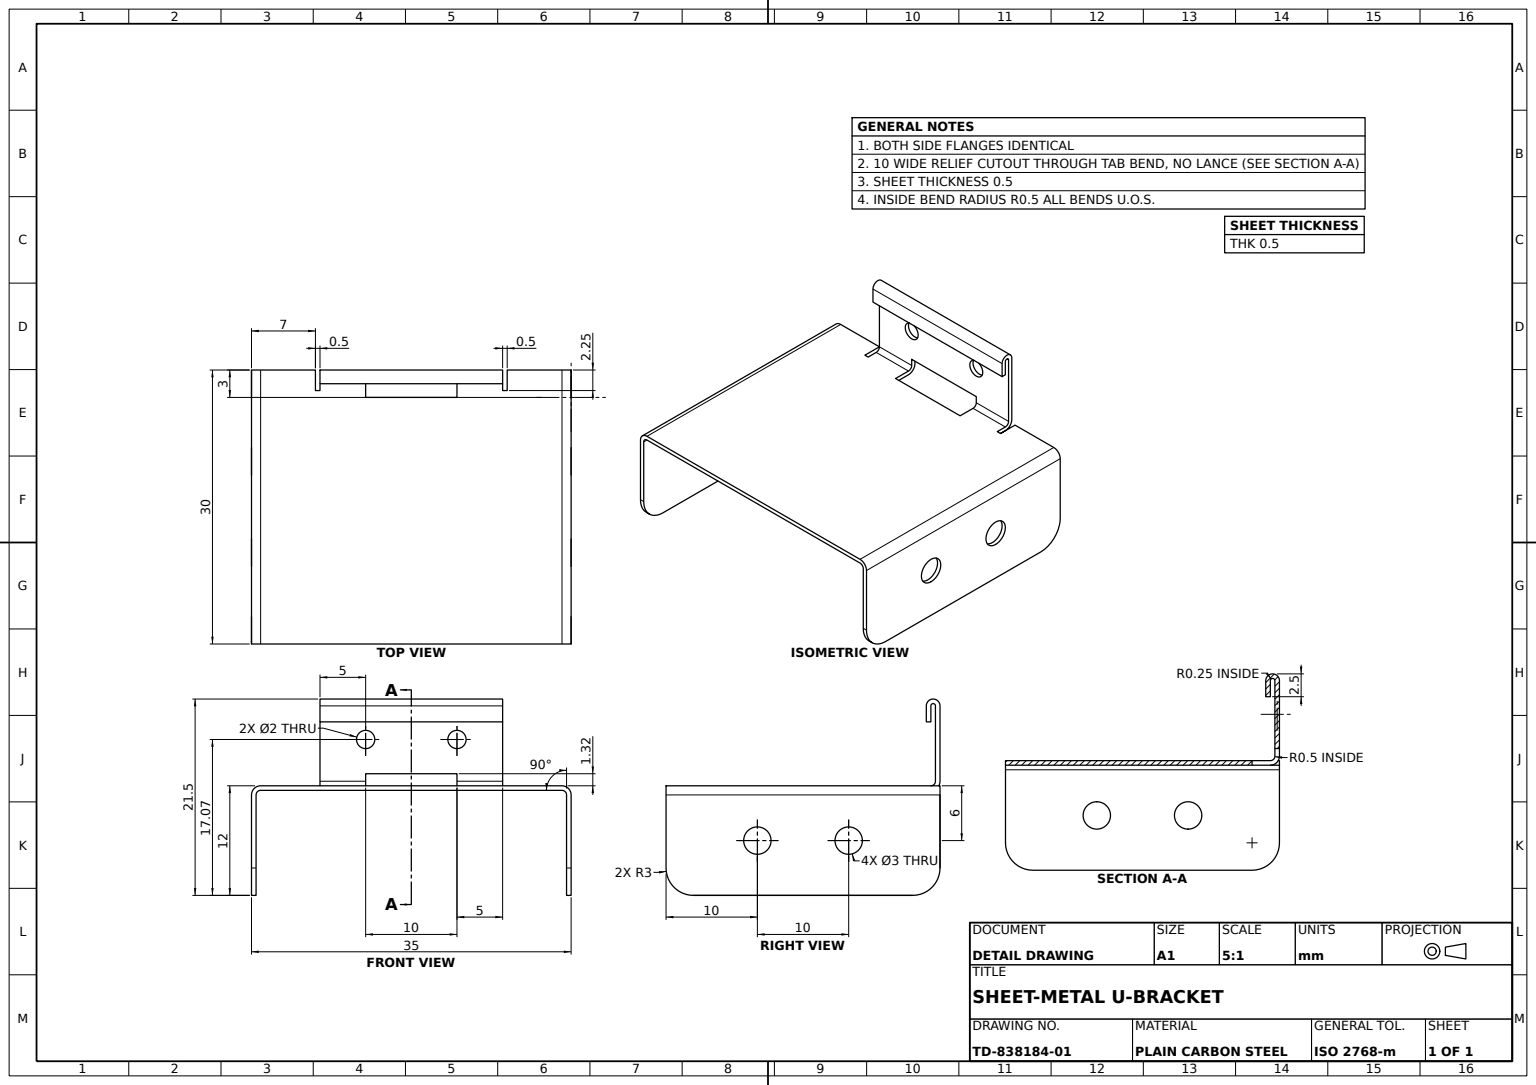
solid
v1 (-17.5,-1,-15)
v2 (-17.5,-9,-15)
e1 v1 v2 LINE
v3 (-17,-1,-15)
e2 v3 v1 LINE
v4 (-17,-9,-15)
e3 v3 v4 LINE
e4 v4 v2 LINE
face PLANE(AX(P(-17.5,-12,-15),D(0,0,1),D(1,0,0))) rev [-e1 -e2 e3 e4]
v5 (17.5,-9,-15)
v6 (17,-9,-15)
e5 v5 v6 LINE
v7 (17,-1,-15)
e6 v6 v7 LINE
v8 (17.5,-1,-15)
e7 v7 v8 LINE
e8 v5 v8 LINE
face PLANE(AX(P(17.5,-0.5,-15),D(0,0,1),D(1,0,0))) rev [e5 e6 e7 -e8]
v9 (-10,0,-12.75)
v10 (-10,-0.5,-12.75)
e9 v9 v10 LINE
v11 (-10,0,-14)
e10 v9 v11 LINE
v12 (-10,-0.5,-14)
e11 v11 v12 LINE
e12 v10 v12 LINE
face PLANE(AX(P(-10,0,-12.75),D(-1,0,0),D(0,0,1))) [-e9 e10 e11 -e12]
v13 (-5,1.321903,-15)
v14 (-5,0.5,-15)
e13 v13 v14 LINE
v15 (-5,1.321903,-14.5)
e14 v13 v15 LINE
v16 (-5,0.5,-14.5)
e15 v15 v16 LINE
e16 v14 v16 LINE
face PLANE(AX(P(-5,-2.678097,-15),D(-1,0,0),D(0,-1,0))) rev [-e13 e14 e15 -e16]
v17 (-10,0.5,-14.5)
v18 (-10,8.75,-14.5)
e17 v17 v18 LINE
v19 (-10,8.75,-15)
e18 v18 v19 LINE
v20 (-10,0.5,-15)
e19 v20 v19 LINE
e20 v17 v20 LINE
face PLANE(AX(P(-10,9.5,-15),D(1,0,0),D(0,0,-1))) rev [e17 e18 -e19 -e20]
v21 (16.5,-0.5,-15)
e21 v21 v7 CIRCLE(AX(P(16.5,-1,-15),D(0,0,-1),D(-1,0,0)),0.5)
v22 (17,-1,15)
e22 v7 v22 LINE
v23 (16.5,-0.5,15)
e23 v22 v23 CIRCLE(AX(P(16.5,-1,15),D(0,0,1),D(1,0,0)),0.5)
e24 v23 v21 LINE
face CYL(AX(P(16.5,-1,-30.027286),D(0,0,1),D(1,0,0)),0.5) rev [e21 e22 e23 e24]
v24 (5,4.070796,-15)
v25 (5,4.070796,-14.5)
e25 v24 v25 LINE
v26 (5,6.070796,-14.5)
e26 v25 v26 CIRCLE(AX(P(5,5.070796,-14.5),D(0,0,1),D(0,1,0)),1)
v27 (5,6.070796,-15)
e27 v27 v26 LINE
e28 v24 v27 CIRCLE(AX(P(5,5.070796,-15),D(0,0,1),D(0,1,0)),1)
face CYL(AX(P(5,5.070796,-15),D(0,0,1),D(0,-1,0)),1) rev [e25 e26 -e27 -e28]
v28 (5,1.321903,-15)
e29 v28 v13 LINE
v29 (5,1.321903,-14.5)
e30 v28 v29 LINE
e31 v29 v15 LINE
face PLANE(AX(P(-5,1.321903,-15),D(0,1,0),D(-1,0,0))) rev [-e14 -e29 e30 e31]
v30 (17,-7.5,5)
v31 (17.5,-7.5,5)
e32 v30 v31 LINE
v32 (17,-4.5,5)
e33 v30 v32 CIRCLE(AX(P(17,-6,5),D(-1,0,0),D(0,-1,0)),1.5)
v33 (17.5,-4.5,5)
e34 v32 v33 LINE
e35 v33 v31 CIRCLE(AX(P(17.5,-6,5),D(1,0,0),D(0,-1,0)),1.5)
face CYL(AX(P(-17.5,-6,5),D(1,0,0),D(0,1,0)),1.5) rev [-e32 e33 e34 e35]
v34 (-5,-0.5,-14)
e36 v14 v34 CIRCLE(AX(P(-5,0.5,-14),D(-1,0,0),D(0,0,1)),1)
e37 v12 v34 LINE
e38 v12 v20 CIRCLE(AX(P(-10,0.5,-14),D(1,0,0),D(0,0,-1)),1)
e39 v20 v14 LINE
face CYL(AX(P(-12.661193,0.5,-14),D(1,0,0),D(0,1,0)),1) [e36 -e37 e38 e39]
v35 (16.5,0,-15)
e40 v21 v35 LINE
e41 v35 v8 CIRCLE(AX(P(16.5,-1,-15),D(0,0,-1),D(1,0,0)),1)
face PLANE(AX(P(16.5,-1,-15),D(0,0,1),D(1,0,0))) rev [-e21 e40 e41 -e7]
e42 v11 v17 CIRCLE(AX(P(-10,0.5,-14),D(1,0,0),D(0,1,0)),0.5)
face PLANE(AX(P(-10,0.5,-14),D(-1,0,0),D(0,0,1))) [-e38 -e11 e42 e20]
v36 (16.5,0,15)
e43 v23 v36 LINE
v37 (17.5,-1,15)
e44 v22 v37 LINE
e45 v37 v36 CIRCLE(AX(P(16.5,-1,15),D(0,0,1),D(1,0,0)),1)
face PLANE(AX(P(16.5,-1,15),D(0,0,-1),D(-1,0,0))) rev [-e43 -e23 e44 e45]
v38 (10,-0.5,-12.75)
v39 (10.5,-0.5,-12.75)
e46 v38 v39 LINE
v40 (10,0,-12.75)
e47 v40 v38 LINE
v41 (10.5,0,-12.75)
e48 v40 v41 LINE
e49 v41 v39 LINE
face PLANE(AX(P(10,0,-12.75),D(0,0,-1),D(0,1,0))) [-e46 -e47 e48 e49]
v42 (-10.5,0,-15)
v43 (-10.5,-0.5,-15)
e50 v42 v43 LINE
v44 (-16.5,-0.5,-15)
e51 v43 v44 LINE
v45 (-16.5,0,-15)
e52 v44 v45 LINE
e53 v42 v45 LINE
face PLANE(AX(P(-17.5,-0.5,-15),D(0,0,-1),D(-1,0,0))) [e50 e51 e52 -e53]
v46 (10,8.75,-13.5)
v47 (10,7,-13.5)
e54 v46 v47 LINE
v48 (-10,8.75,-13.5)
e55 v48 v46 LINE
v49 (-10,7,-13.5)
e56 v49 v48 LINE
e57 v47 v49 LINE
face PLANE(AX(P(0,7.875,-13.5),D(0,0,1),D(0,-1,0))) [-e54 -e55 -e56 -e57]
v50 (10,7,-14)
v51 (-10,7,-14)
e58 v50 v51 LINE
v52 (-10,8.75,-14)
e59 v51 v52 LINE
v53 (10,8.75,-14)
e60 v52 v53 LINE
e61 v53 v50 LINE
face PLANE(AX(P(0,7.875,-14),D(0,0,1),D(0,-1,0))) rev [e58 e59 e60 e61]
v54 (10,0,-14)
v55 (10,-0.5,-14)
e62 v54 v55 LINE
e63 v54 v40 LINE
e64 v55 v38 LINE
face PLANE(AX(P(10,0,-14),D(1,0,0),D(0,0,-1))) [-e62 e63 e47 -e64]
v56 (5,0,-14)
e65 v56 v54 LINE
v57 (5,0,-12)
e66 v57 v56 LINE
v58 (-5,0,-12)
e67 v58 v57 LINE
v59 (-5,0,-14)
e68 v59 v58 LINE
e69 v11 v59 LINE
v60 (-10.5,0,-12.75)
e70 v60 v9 LINE
e71 v42 v60 LINE
v61 (-16.5,0,15)
e72 v45 v61 LINE
e73 v61 v36 LINE
e74 v36 v35 LINE
v62 (10.5,0,-15)
e75 v35 v62 LINE
e76 v41 v62 LINE
face PLANE(AX(P(0,0,0),D(0,-1,0),D(0,0,-1))) rev [-e63 -e65 -e66 -e67 -e68 -e69 -e10 -e70 -e71 e53 e72 e73 e74 e75 -e76 -e48]
v63 (-17.5,-9,15)
v64 (-17,-9,15)
e77 v63 v64 LINE
v65 (-17.5,-12,12)
e78 v65 v63 CIRCLE(AX(P(-17.5,-9,12),D(-1,0,0),D(0,1,0)),3)
v66 (-17,-12,12)
e79 v66 v65 LINE
e80 v64 v66 CIRCLE(AX(P(-17,-9,12),D(1,0,0),D(0,1,0)),3)
face CYL(AX(P(-17.5,-9,12),D(1,0,0),D(0,1,0)),3) [-e77 -e78 -e79 -e80]
v67 (17.5,-7.5,-5)
v68 (17.5,-4.5,-5)
e81 v67 v68 CIRCLE(AX(P(17.5,-6,-5),D(1,0,0),D(0,1,0)),1.5)
v69 (17,-4.5,-5)
e82 v69 v68 LINE
v70 (17,-7.5,-5)
e83 v69 v70 CIRCLE(AX(P(17,-6,-5),D(-1,0,0),D(0,-1,0)),1.5)
e84 v70 v67 LINE
face CYL(AX(P(-17.5,-6,-5),D(1,0,0),D(0,1,0)),1.5) rev [e81 -e82 e83 e84]
v71 (-5,-0.5,-12)
v72 (5,-0.5,-12)
e85 v71 v72 LINE
e86 v71 v58 LINE
e87 v72 v57 LINE
face PLANE(AX(P(-5,-0.5,-12),D(0,0,1),D(1,0,0))) rev [-e85 e86 e67 -e87]
v73 (-10.5,-0.5,-12.75)
e88 v73 v10 LINE
e89 v60 v73 LINE
face PLANE(AX(P(-10.5,0,-12.75),D(0,0,-1),D(0,1,0))) [e9 -e88 -e89 e70]
e90 v32 v30 CIRCLE(AX(P(17,-6,5),D(-1,0,0),D(0,-1,0)),1.5)
e91 v31 v33 CIRCLE(AX(P(17.5,-6,5),D(1,0,0),D(0,-1,0)),1.5)
face CYL(AX(P(-17.5,-6,5),D(1,0,0),D(0,1,0)),1.5) rev [-e34 e90 e32 e91]
e92 v26 v25 CIRCLE(AX(P(5,5.070796,-14.5),D(0,0,1),D(0,1,0)),1)
e93 v27 v24 CIRCLE(AX(P(5,5.070796,-15),D(0,0,1),D(0,1,0)),1)
face CYL(AX(P(5,5.070796,-15),D(0,0,1),D(0,-1,0)),1) rev [e27 e92 -e25 -e93]
v74 (-5,4.070796,-15)
v75 (-5,6.070796,-15)
e94 v74 v75 CIRCLE(AX(P(-5,5.070796,-15),D(0,0,1),D(0,-1,0)),1)
v76 (-5,4.070796,-14.5)
e95 v74 v76 LINE
v77 (-5,6.070796,-14.5)
e96 v76 v77 CIRCLE(AX(P(-5,5.070796,-14.5),D(0,0,1),D(0,-1,0)),1)
e97 v75 v77 LINE
face CYL(AX(P(-5,5.070796,-15),D(0,0,1),D(0,-1,0)),1) rev [-e94 e95 e96 -e97]
e98 v77 v76 CIRCLE(AX(P(-5,5.070796,-14.5),D(0,0,1),D(0,-1,0)),1)
v78 (5,0.5,-14.5)
e99 v78 v29 LINE
v79 (10,0.5,-14.5)
e100 v79 v78 LINE
v80 (10,8.75,-14.5)
e101 v80 v79 LINE
e102 v18 v80 LINE
e103 v16 v17 LINE
face PLANE(AX(P(0,0,-14.5),D(0,0,1),D(0,-1,0))) [-e92 -e26] [-e96 -e98] [-e99 -e100 -e101 -e102 -e17 -e103 -e15 -e31]
v81 (17,-12,12)
v82 (17,-9,15)
e104 v81 v82 CIRCLE(AX(P(17,-9,12),D(-1,0,0),D(0,-1,0)),3)
e105 v22 v82 LINE
v83 (17,-12,-12)
e106 v6 v83 CIRCLE(AX(P(17,-9,-12),D(-1,0,0),D(0,-1,0)),3)
e107 v81 v83 LINE
e108 v70 v69 CIRCLE(AX(P(17,-6,-5),D(-1,0,0),D(0,-1,0)),1.5)
face PLANE(AX(P(17,0,0),D(-1,0,0),D(0,-1,0))) [e104 -e105 -e22 -e6 e106 -e107] [-e108 -e83] [-e90 -e33]
v84 (10.5,-0.5,-15)
e109 v21 v84 LINE
e110 v62 v84 LINE
face PLANE(AX(P(-17.5,-0.5,-15),D(0,0,-1),D(-1,0,0))) [-e75 -e40 e109 -e110]
e111 v75 v74 CIRCLE(AX(P(-5,5.070796,-15),D(0,0,1),D(0,-1,0)),1)
face CYL(AX(P(-5,5.070796,-15),D(0,0,1),D(0,-1,0)),1) rev [-e95 -e111 e97 e98]
v85 (5,-0.5,-14)
v86 (5,0.5,-15)
e112 v85 v86 CIRCLE(AX(P(5,0.5,-14),D(1,0,0),D(0,0,-1)),1)
e113 v85 v56 LINE
e114 v56 v78 CIRCLE(AX(P(5,0.5,-14),D(1,0,0),D(0,1,0)),0.5)
e115 v78 v86 LINE
face PLANE(AX(P(5,0.5,-14),D(-1,0,0),D(0,0,1))) [-e112 e113 e114 e115]
v87 (-17.5,-4.5,-5)
v88 (-17.5,-7.5,-5)
e116 v87 v88 CIRCLE(AX(P(-17.5,-6,-5),D(1,0,0),D(0,1,0)),1.5)
v89 (-17,-4.5,-5)
e117 v87 v89 LINE
v90 (-17,-7.5,-5)
e118 v89 v90 CIRCLE(AX(P(-17,-6,-5),D(1,0,0),D(0,1,0)),1.5)
e119 v88 v90 LINE
face CYL(AX(P(-17.5,-6,-5),D(1,0,0),D(0,1,0)),1.5) rev [-e116 e117 e118 -e119]
e120 v86 v28 LINE
face PLANE(AX(P(5,-2.678097,-15),D(1,0,0),D(0,1,0))) rev [-e115 e99 -e30 -e120]
e121 v16 v59 CIRCLE(AX(P(-5,0.5,-14),D(-1,0,0),D(0,1,0)),0.5)
e122 v59 v34 LINE
face PLANE(AX(P(-5,0.5,-14),D(1,0,0),D(0,0,-1))) [e16 e121 e122 -e36]
v91 (17.5,-9,15)
e123 v82 v91 LINE
e124 v37 v91 LINE
face PLANE(AX(P(17.5,-12,15),D(0,0,-1),D(-1,0,0))) rev [e123 -e124 -e44 e105]
v92 (-17.5,-4.5,5)
v93 (-17.5,-7.5,5)
e125 v92 v93 CIRCLE(AX(P(-17.5,-6,5),D(1,0,0),D(0,-1,0)),1.5)
v94 (-17,-4.5,5)
e126 v92 v94 LINE
v95 (-17,-7.5,5)
e127 v94 v95 CIRCLE(AX(P(-17,-6,5),D(1,0,0),D(0,1,0)),1.5)
e128 v93 v95 LINE
face CYL(AX(P(-17.5,-6,5),D(1,0,0),D(0,1,0)),1.5) rev [-e125 e126 e127 -e128]
e129 v1 v45 CIRCLE(AX(P(-16.5,-1,-15),D(0,0,-1),D(-1,0,0)),1)
v96 (-17.5,-1,15)
e130 v1 v96 LINE
e131 v61 v96 CIRCLE(AX(P(-16.5,-1,15),D(0,0,1),D(-1,0,0)),1)
face CYL(AX(P(-16.5,-1,30.027286),D(0,0,-1),D(-1,0,0)),1) [-e72 -e129 e130 -e131]
v97 (10,0.5,-15)
e132 v97 v55 CIRCLE(AX(P(10,0.5,-14),D(-1,0,0),D(0,0,1)),1)
e133 v79 v97 LINE
e134 v79 v54 CIRCLE(AX(P(10,0.5,-14),D(-1,0,0),D(0,1,0)),0.5)
face PLANE(AX(P(10,0.5,-14),D(1,0,0),D(0,0,-1))) [e62 -e132 -e133 e134]
e135 v37 v8 LINE
face CYL(AX(P(16.5,-1,-30.027286),D(0,0,1),D(1,0,0)),1) [-e74 -e45 e135 -e41]
e136 v86 v97 LINE
e137 v85 v55 LINE
face CYL(AX(P(2.338807,0.5,-14),D(1,0,0),D(0,1,0)),1) [e112 e136 e132 -e137]
e138 v34 v71 LINE
face PLANE(AX(P(-5,-0.5,-12),D(-1,0,0),D(0,0,1))) rev [-e138 -e122 e68 -e86]
e139 v95 v94 CIRCLE(AX(P(-17,-6,5),D(1,0,0),D(0,1,0)),1.5)
e140 v93 v92 CIRCLE(AX(P(-17.5,-6,5),D(1,0,0),D(0,-1,0)),1.5)
face CYL(AX(P(-17.5,-6,5),D(1,0,0),D(0,1,0)),1.5) rev [e128 e139 -e126 -e140]
e141 v90 v89 CIRCLE(AX(P(-17,-6,-5),D(1,0,0),D(0,1,0)),1.5)
e142 v88 v87 CIRCLE(AX(P(-17.5,-6,-5),D(1,0,0),D(0,1,0)),1.5)
face CYL(AX(P(-17.5,-6,-5),D(1,0,0),D(0,1,0)),1.5) rev [e141 -e117 -e142 e119]
e143 v3 v44 CIRCLE(AX(P(-16.5,-1,-15),D(0,0,-1),D(-1,0,0)),0.5)
face PLANE(AX(P(-16.5,-1,-15),D(0,0,1),D(1,0,0))) rev [e2 e129 -e52 -e143]
v98 (17.5,-12,12)
e144 v98 v81 LINE
v99 (17.5,-12,-12)
e145 v83 v99 LINE
e146 v98 v99 LINE
face PLANE(AX(P(17.5,-12,-15),D(0,1,0),D(-1,0,0))) rev [e144 e107 e145 -e146]
v100 (-16.5,-0.5,15)
e147 v100 v61 LINE
e148 v100 v23 LINE
face PLANE(AX(P(-17.5,-0.5,15),D(0,0,1),D(1,0,0))) [e43 -e73 -e147 e148]
e149 v68 v67 CIRCLE(AX(P(17.5,-6,-5),D(1,0,0),D(0,1,0)),1.5)
face CYL(AX(P(-17.5,-6,-5),D(1,0,0),D(0,1,0)),1.5) rev [e149 -e84 e108 e82]
e150 v91 v98 CIRCLE(AX(P(17.5,-9,12),D(1,0,0),D(0,-1,0)),3)
face CYL(AX(P(17.5,-9,12),D(-1,0,0),D(0,-1,0)),3) [-e104 -e144 -e150 -e123]
v101 (10,8.75,-15)
e151 v19 v101 LINE
e152 v101 v97 LINE
face PLANE(AX(P(0,0,-15),D(0,0,1),D(0,-1,0))) rev [e28 e93] [-e136 e120 e29 e13 -e39 e19 e151 e152] [e94 e111]
v102 (-17,-1,15)
e153 v102 v3 LINE
e154 v44 v100 LINE
e155 v100 v102 CIRCLE(AX(P(-16.5,-1,15),D(0,0,1),D(1,0,0)),0.5)
face CYL(AX(P(-16.5,-1,30.027286),D(0,0,-1),D(-1,0,0)),0.5) rev [e153 e143 e154 e155]
e156 v50 v47 LINE
e157 v51 v49 LINE
face PLANE(AX(P(0,7,-13.5),D(0,1,0),D(-1,0,0))) rev [e156 e57 -e157 -e58]
e158 v72 v85 LINE
e159 v39 v84 LINE
e160 v43 v73 LINE
face PLANE(AX(P(0,-0.5,0),D(0,-1,0),D(0,0,-1))) [e12 e37 e138 e85 e158 e137 e64 e46 e159 -e109 -e24 -e148 -e154 -e51 e160 e88]
face CYL(AX(P(2.338807,0.5,-14),D(1,0,0),D(0,1,0)),0.5) rev [-e114 e65 -e134 e100]
e161 v102 v96 LINE
e162 v63 v96 LINE
e163 v64 v102 LINE
face PLANE(AX(P(-17.5,-0.5,15),D(0,0,-1),D(-1,0,0))) rev [e161 -e162 e77 e163]
e164 v53 v80 CIRCLE(AX(P(10,8.75,-14.25),D(-1,0,0),D(0,0,1)),0.25)
e165 v80 v101 LINE
e166 v46 v101 CIRCLE(AX(P(10,8.75,-14.25),D(-1,0,0),D(0,-1,0)),0.75)
e167 v53 v46 LINE
face PLANE(AX(P(10,8.75,-14.25),D(1,0,0),D(0,1,0))) [e164 e165 -e166 -e167]
v103 (-17,-12,-12)
e168 v103 v66 LINE
e169 v103 v4 CIRCLE(AX(P(-17,-9,-12),D(1,0,0),D(0,1,0)),3)
face PLANE(AX(P(-17,0,0),D(1,0,0),D(0,1,0))) [-e141 -e118] [-e3 -e153 -e163 e80 -e168 e169] [-e127 -e139]
face PLANE(AX(P(-10.5,0,-15),D(1,0,0),D(0,0,-1))) [-e50 e71 e89 -e160]
face CYL(AX(P(-12.661193,0.5,-14),D(1,0,0),D(0,1,0)),0.5) rev [-e42 e69 -e121 e103]
e170 v18 v52 CIRCLE(AX(P(-10,8.75,-14.25),D(1,0,0),D(0,0,1)),0.25)
face CYL(AX(P(-20.06782,8.75,-14.25),D(1,0,0),D(0,0,1)),0.25) rev [e102 -e164 -e60 -e170]
v104 (-17.5,-12,-12)
e171 v104 v103 LINE
e172 v2 v104 CIRCLE(AX(P(-17.5,-9,-12),D(-1,0,0),D(0,1,0)),3)
face CYL(AX(P(-17.5,-9,-12),D(1,0,0),D(0,1,0)),3) [-e171 -e172 -e4 -e169]
face PLANE(AX(P(10,7.875,-13.5),D(-1,0,0),D(0,-1,0))) rev [e54 -e156 -e61 e167]
face PLANE(AX(P(-16.5,-1,15),D(0,0,-1),D(-1,0,0))) rev [-e155 e147 e131 -e161]
face PLANE(AX(P(5,-0.5,-12),D(1,0,0),D(0,0,-1))) rev [-e113 -e158 e87 e66]
e173 v99 v5 CIRCLE(AX(P(17.5,-9,-12),D(1,0,0),D(0,-1,0)),3)
face CYL(AX(P(17.5,-9,-12),D(-1,0,0),D(0,-1,0)),3) [-e106 -e5 -e173 -e145]
e174 v104 v65 LINE
face PLANE(AX(P(-17.5,-12,15),D(0,1,0),D(-1,0,0))) rev [e79 -e174 e171 e168]
e175 v52 v48 LINE
face PLANE(AX(P(-10,7.875,-13.5),D(1,0,0),D(0,1,0))) rev [-e175 -e59 e157 e56]
e176 v19 v48 CIRCLE(AX(P(-10,8.75,-14.25),D(1,0,0),D(0,1,0)),0.75)
face PLANE(AX(P(-10,8.75,-14.25),D(-1,0,0),D(0,-1,0))) [e175 -e176 -e18 e170]
face PLANE(AX(P(10,0,-15),D(-1,0,0),D(0,-1,0))) rev [-e152 -e165 e101 e133]
face CYL(AX(P(-20.06782,8.75,-14.25),D(1,0,0),D(0,0,1)),0.75) [-e151 e176 e55 e166]
face PLANE(AX(P(17.5,0,0),D(-1,0,0),D(0,-1,0))) rev [e8 -e135 e124 e150 e146 e173] [-e35 -e91] [-e149 -e81]
face PLANE(AX(P(10.5,0,-12.75),D(-1,0,0),D(0,0,1))) [e110 -e159 -e49 e76]
face PLANE(AX(P(-17.5,0,0),D(1,0,0),D(0,1,0))) rev [e172 e174 e78 e162 -e130 e1] [e142 e116] [e140 e125]
